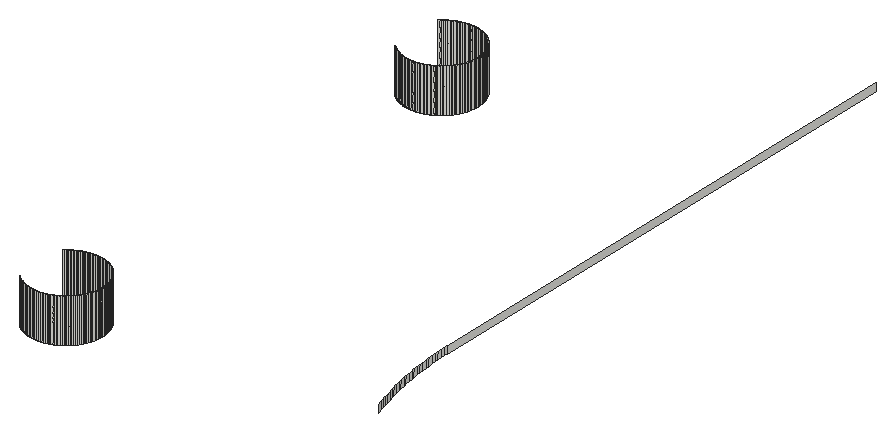
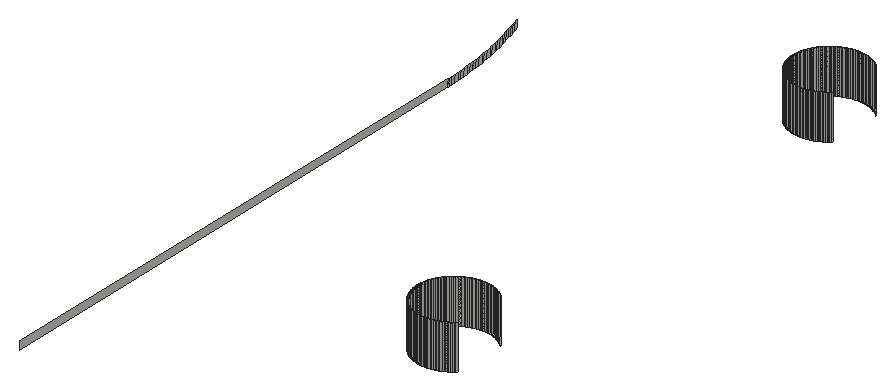
# SketchUp Ruby script. Lengths in inches.
U = 1.inch
M = Sketchup.active_model
def pt(a) = Geom::Point3d.new(a.map { |v| v * U })
def face(e, loops, mat)
  f = e.add_face(loops[0].map { |a| pt(a) })
  loops[1..].each { |l| e.add_face(l.map { |a| pt(a) }).erase! }
  f.material = f.back_material = mat if mat
  f
end
# faces: each face lists its corners as indices into pts; further lists are holes
def faces(e, pts, list, mat = nil) = list.each { |f| face(e, (f[0].is_a?(Array) ? f : [f]).map { |l| l.map { |i| pts[i] } }, mat) }
# xy, xz, yz: faces in a plane at the given z, y or x. An outline is a flat list of corners, or four numbers for a rectangle; further outlines are holes
def ring(l) = l.size == 4 ? [[l[0], l[1]], [l[2], l[1]], [l[2], l[3]], [l[0], l[3]]] : l.each_slice(2).to_a
def flat(e, list, mat, &to3) = list.each { |f| face(e, (f[0].is_a?(Array) ? f : [f]).map { |l| ring(l).map { |u, v| to3.(u, v) } }, mat) }
def xy(e, z, list, mat = nil) = flat(e, list, mat) { |x, y| [x, y, z] }
def xz(e, y, list, mat = nil) = flat(e, list, mat) { |x, z| [x, y, z] }
def yz(e, x, list, mat = nil) = flat(e, list, mat) { |y, z| [x, y, z] }
def lines(e, pts, list) = list.each { |a, b| e.add_line(pt(pts[a]), pt(pts[b])) }
# prism: a flat outline (further loops are holes) pulled along v
def prism(e, loops, v, mat = nil)
  f = face(e, loops, mat); d = Geom::Vector3d.new(v.map { |x| x * U })
  f.pushpull(f.normal.samedirection?(d) ? d.length : -d.length)
end
def box(e, o, s, mat = nil) = prism(e, [[o, [o[0] + s[0], o[1], o[2]], [o[0] + s[0], o[1] + s[1], o[2]], [o[0], o[1] + s[1], o[2]]]], [0, 0, s[2]], mat)
def at(x, y, z, deg = 0) = Geom::Transformation.translation(pt([x, y, z])) * Geom::Transformation.rotation(ORIGIN, Z_AXIS, deg.degrees)
def axes(o, x, y, z) = Geom::Transformation.new([*x, 0, *y, 0, *z, 0, *pt(o).to_a, 1])
def part(name) = M.definitions.add(name)
# library, detail: a bought-in or finely detailed component or shape, given as its bounding box
def library(name, o, s) = part(name).tap { |d| box(d.entities, o, s) }
def detail(e, o, s) = box(e.add_group.entities, o, s)
def put(e, d, t, mat = nil) = e.add_instance(d, t).tap { |i| i.material = mat if mat }
def group(e, t, mat = nil) = e.add_group.tap { |g| g.transformation = t; g.material = mat if mat }.entities
root = M.entities
xz(root,197.5,[[110.34,116,110.42,119],[110.42,116,110.5,119],[110.5,116,110.58,119],[110.58,116,110.66,119]])
xz(root,202.5,[[110.34,116,110.42,119],[110.42,116,110.5,119],[110.5,116,110.58,119],[110.58,116,110.66,119]])
xz(root,229.5,[[110.34,116,110.42,119],[110.42,116,110.5,119],[110.5,116,110.58,119],[110.58,116,110.66,119]])
xz(root,234.5,[[110.34,116,110.42,119],[110.42,116,110.5,119],[110.5,116,110.58,119],[110.58,116,110.66,119]])
yz(root,113,[[199.84,116,199.92,119],[199.92,116,200,119],[200,116,200.08,119],[200.08,116,200.16,119],[231.84,116,231.92,119],
  [231.92,116,232,119],[232,116,232.08,119],[232.08,116,232.16,119]])
yz(root,128.5,[[209.72,116,209.95,116.5],[209.95,116,209.99,116.5],[209.99,116,246.5,116.5]])
p = [[110.03,197.54,116],[109.95,197.56,116],[109.95,197.56,119],[110.03,197.54,119],[110.11,197.53,116],[110.11,197.53,119],
  [110.1875,197.52,116],[110.1875,197.52,119],[110.26,197.51,116],[110.26,197.51,119],[110.34,197.5,116],[110.34,197.5,119],
  [110.74,197.51,116],[110.66,197.5,116],[110.66,197.5,119],[110.74,197.51,119],[110.8125,197.52,116],[110.8125,197.52,119],
  [110.89,197.53,116],[110.89,197.53,119],[110.97,197.54,116],[110.97,197.54,119],[111.05,197.56,116],[111.05,197.56,119],
  [109.65,197.65,116],[109.58,197.68,116],[109.58,197.68,119],[109.65,197.65,119],[109.73,197.62,116],[109.73,197.62,119],
  [109.8,197.6,116],[109.8,197.6,119],[109.88,197.58,116],[109.88,197.58,119],[111.12,197.58,116],[111.12,197.58,119],
  [111.2,197.6,116],[111.2,197.6,119],[111.27,197.62,116],[111.27,197.62,119],[111.35,197.65,116],[111.35,197.65,119],
  [111.42,197.68,116],[111.42,197.68,119],[109.4375,197.74,116],[109.37,197.77,116],[109.37,197.77,119],[109.4375,197.74,119],
  [109.51,197.71,116],[109.51,197.71,119],[111.49,197.71,116],[111.49,197.71,119],[111.5625,197.74,116],[111.5625,197.74,119],
  [111.63,197.77,116],[111.63,197.77,119],[109.23,197.85,116],[109.16,197.89,116],[109.16,197.89,119],[109.23,197.85,119],
  [109.3,197.81,116],[109.3,197.81,119],[111.7,197.81,116],[111.7,197.81,119],[111.77,197.85,116],[111.77,197.85,119],
  [111.84,197.89,116],[111.84,197.89,119],[109.09,197.93,116],[109.03,197.98,116],[109.03,197.98,119],[109.09,197.93,119],
  [111.91,197.93,116],[111.91,197.93,119],[111.97,197.98,116],[111.97,197.98,119],[108.97,198.02,116],[108.91,198.07,116],
  [108.91,198.07,119],[108.97,198.02,119],[112.03,198.02,116],[112.03,198.02,119],[112.09,198.07,116],[112.09,198.07,119],
  [108.85,198.125,116],[108.79,198.18,116],[108.79,198.18,119],[108.85,198.125,119],[112.15,198.125,116],[112.15,198.125,119],
  [112.21,198.18,116],[112.21,198.18,119],[112.27,198.23,116],[112.27,198.23,119],[112.32,198.29,116],[112.32,198.29,119],
  [112.375,198.35,116],[112.375,198.35,119],[112.43,198.41,116],[112.43,198.41,119],[112.48,198.47,116],[112.48,198.47,119],
  [112.52,198.53,116],[112.52,198.53,119],[112.57,198.59,116],[112.57,198.59,119],[112.61,198.66,116],[112.61,198.66,119],
  [112.65,198.73,116],[112.65,198.73,119],[112.69,198.8,116],[112.69,198.8,119],[112.73,198.87,116],[112.73,198.87,119],
  [112.76,198.9375,116],[112.76,198.9375,119],[112.79,199.01,116],[112.79,199.01,119],[112.82,199.08,116],[112.82,199.08,119],
  [112.85,199.15,116],[112.85,199.15,119],[112.88,199.23,116],[112.88,199.23,119],[112.9,199.3,116],[112.9,199.3,119],
  [112.92,199.38,116],[112.92,199.38,119],[112.94,199.45,116],[112.94,199.45,119],[112.96,199.53,116],[112.96,199.53,119],
  [112.97,199.61,116],[112.97,199.61,119],[112.98,199.6875,116],[112.98,199.6875,119],[112.99,199.76,116],[112.99,199.76,119],
  [113,199.84,116],[113,199.84,119],[112.98,200.3125,116],[112.99,200.24,116],[112.99,200.24,119],[112.98,200.3125,119],
  [113,200.16,116],[113,200.16,119],[112.97,200.39,116],[112.97,200.39,119],[112.96,200.47,116],[112.96,200.47,119],
  [112.92,200.62,116],[112.94,200.55,116],[112.94,200.55,119],[112.92,200.62,119],[112.9,200.7,116],[112.9,200.7,119],
  [112.88,200.77,116],[112.88,200.77,119],[112.82,200.92,116],[112.85,200.85,116],[112.85,200.85,119],[112.82,200.92,119],
  [112.79,200.99,116],[112.79,200.99,119],[112.76,201.0625,116],[112.76,201.0625,119],[112.69,201.2,116],[112.73,201.13,116],
  [112.73,201.13,119],[112.69,201.2,119],[112.65,201.27,116],[112.65,201.27,119],[112.57,201.41,116],[112.61,201.34,116],
  [112.61,201.34,119],[112.57,201.41,119],[112.52,201.47,116],[112.52,201.47,119],[112.43,201.59,116],[112.48,201.53,116],
  [112.48,201.53,119],[112.43,201.59,119],[112.375,201.65,116],[112.375,201.65,119],[112.27,201.77,116],[112.32,201.71,116],
  [112.32,201.71,119],[112.27,201.77,119],[108.79,201.82,116],[108.85,201.875,116],[108.85,201.875,119],[108.79,201.82,119],
  [112.15,201.875,116],[112.21,201.82,116],[112.21,201.82,119],[112.15,201.875,119],[108.91,201.93,116],[108.91,201.93,119],
  [108.97,201.98,116],[108.97,201.98,119],[112.03,201.98,116],[112.09,201.93,116],[112.09,201.93,119],[112.03,201.98,119],
  [109.03,202.02,116],[109.03,202.02,119],[109.09,202.07,116],[109.09,202.07,119],[111.91,202.07,116],[111.97,202.02,116],
  [111.97,202.02,119],[111.91,202.07,119],[109.16,202.11,116],[109.16,202.11,119],[109.23,202.15,116],[109.23,202.15,119],
  [111.77,202.15,116],[111.84,202.11,116],[111.84,202.11,119],[111.77,202.15,119],[109.3,202.19,116],[109.3,202.19,119],
  [109.37,202.23,116],[109.37,202.23,119],[109.4375,202.26,116],[109.4375,202.26,119],[111.5625,202.26,116],[111.63,202.23,116],
  [111.63,202.23,119],[111.5625,202.26,119],[111.7,202.19,116],[111.7,202.19,119],[109.51,202.29,116],[109.51,202.29,119],
  [109.58,202.32,116],[109.58,202.32,119],[109.65,202.35,116],[109.65,202.35,119],[111.35,202.35,116],[111.42,202.32,116],
  [111.42,202.32,119],[111.35,202.35,119],[111.49,202.29,116],[111.49,202.29,119],[109.73,202.38,116],[109.73,202.38,119],
  [109.8,202.4,116],[109.8,202.4,119],[109.88,202.42,116],[109.88,202.42,119],[109.95,202.44,116],[109.95,202.44,119],
  [110.03,202.46,116],[110.03,202.46,119],[110.97,202.46,116],[111.05,202.44,116],[111.05,202.44,119],[110.97,202.46,119],
  [111.12,202.42,116],[111.12,202.42,119],[111.2,202.4,116],[111.2,202.4,119],[111.27,202.38,116],[111.27,202.38,119],
  [110.11,202.47,116],[110.11,202.47,119],[110.1875,202.48,116],[110.1875,202.48,119],[110.26,202.49,116],[110.26,202.49,119],
  [110.34,202.5,116],[110.34,202.5,119],[110.66,202.5,116],[110.74,202.49,116],[110.74,202.49,119],[110.66,202.5,119],
  [110.8125,202.48,116],[110.8125,202.48,119],[110.89,202.47,116],[110.89,202.47,119],[129.65,202.74,116],[129.5625,203.01,116],
  [129.5625,203.01,116.5],[129.65,202.74,116.5],[129.48,203.28,116],[129.48,203.28,116.5],[129.4,203.55,116],[129.4,203.55,116.5],
  [129.33,203.83,116],[129.33,203.83,116.5],[129.25,204.1,116],[129.25,204.1,116.5],[129.18,204.375,116],[129.18,204.375,116.5],
  [129.12,204.65,116],[129.12,204.65,116.5],[129.05,204.93,116],[129.05,204.93,116.5],[128.99,205.21,116],[128.99,205.21,116.5],
  [128.9375,205.49,116],[128.9375,205.49,116.5],[128.88,205.76,116],[128.88,205.76,116.5],[128.84,206.04,116],[128.84,206.04,116.5],
  [128.79,206.32,116],[128.79,206.32,116.5],[128.75,206.6,116],[128.75,206.6,116.5],[128.71,206.89,116],[128.71,206.89,116.5],
  [128.67,207.17,116],[128.67,207.17,116.5],[128.64,207.45,116],[128.64,207.45,116.5],[128.61,207.73,116],[128.61,207.73,116.5],
  [128.58,208.01,116],[128.58,208.01,116.5],[128.5625,208.3,116],[128.5625,208.3,116.5],[128.54,208.58,116],[128.54,208.58,116.5],
  [128.53,208.86,116],[128.53,208.86,116.5],[128.52,209.15,116],[128.52,209.15,116.5],[128.51,209.43,116],[128.51,209.43,116.5],
  [128.5,209.72,116],[128.5,209.72,116.5],[110.03,229.54,116],[109.95,229.56,116],[109.95,229.56,119],[110.03,229.54,119],
  [110.11,229.53,116],[110.11,229.53,119],[110.1875,229.52,116],[110.1875,229.52,119],[110.26,229.51,116],[110.26,229.51,119],
  [110.34,229.5,116],[110.34,229.5,119],[110.74,229.51,116],[110.66,229.5,116],[110.66,229.5,119],[110.74,229.51,119],
  [110.8125,229.52,116],[110.8125,229.52,119],[110.89,229.53,116],[110.89,229.53,119],[110.97,229.54,116],[110.97,229.54,119],
  [111.05,229.56,116],[111.05,229.56,119],[109.65,229.65,116],[109.58,229.68,116],[109.58,229.68,119],[109.65,229.65,119],
  [109.73,229.62,116],[109.73,229.62,119],[109.8,229.6,116],[109.8,229.6,119],[109.88,229.58,116],[109.88,229.58,119],
  [111.12,229.58,116],[111.12,229.58,119],[111.2,229.6,116],[111.2,229.6,119],[111.27,229.62,116],[111.27,229.62,119],
  [111.35,229.65,116],[111.35,229.65,119],[111.42,229.68,116],[111.42,229.68,119],[109.4375,229.74,116],[109.37,229.77,116],
  [109.37,229.77,119],[109.4375,229.74,119],[109.51,229.71,116],[109.51,229.71,119],[111.49,229.71,116],[111.49,229.71,119],
  [111.5625,229.74,116],[111.5625,229.74,119],[111.63,229.77,116],[111.63,229.77,119],[109.23,229.85,116],[109.16,229.89,116],
  [109.16,229.89,119],[109.23,229.85,119],[109.3,229.81,116],[109.3,229.81,119],[111.7,229.81,116],[111.7,229.81,119],
  [111.77,229.85,116],[111.77,229.85,119],[111.84,229.89,116],[111.84,229.89,119],[109.09,229.93,116],[109.03,229.98,116],
  [109.03,229.98,119],[109.09,229.93,119],[111.91,229.93,116],[111.91,229.93,119],[111.97,229.98,116],[111.97,229.98,119],
  [108.97,230.02,116],[108.91,230.07,116],[108.91,230.07,119],[108.97,230.02,119],[112.03,230.02,116],[112.03,230.02,119],
  [112.09,230.07,116],[112.09,230.07,119],[108.85,230.125,116],[108.79,230.18,116],[108.79,230.18,119],[108.85,230.125,119],
  [112.15,230.125,116],[112.15,230.125,119],[112.21,230.18,116],[112.21,230.18,119],[112.27,230.23,116],[112.27,230.23,119],
  [112.32,230.29,116],[112.32,230.29,119],[112.375,230.35,116],[112.375,230.35,119],[112.43,230.41,116],[112.43,230.41,119],
  [112.48,230.47,116],[112.48,230.47,119],[112.52,230.53,116],[112.52,230.53,119],[112.57,230.59,116],[112.57,230.59,119],
  [112.61,230.66,116],[112.61,230.66,119],[112.65,230.73,116],[112.65,230.73,119],[112.69,230.8,116],[112.69,230.8,119],
  [112.73,230.87,116],[112.73,230.87,119],[112.76,230.9375,116],[112.76,230.9375,119],[112.79,231.01,116],[112.79,231.01,119],
  [112.82,231.08,116],[112.82,231.08,119],[112.85,231.15,116],[112.85,231.15,119],[112.88,231.23,116],[112.88,231.23,119],
  [112.9,231.3,116],[112.9,231.3,119],[112.92,231.38,116],[112.92,231.38,119],[112.94,231.45,116],[112.94,231.45,119],
  [112.96,231.53,116],[112.96,231.53,119],[112.97,231.61,116],[112.97,231.61,119],[112.98,231.6875,116],[112.98,231.6875,119],
  [112.99,231.76,116],[112.99,231.76,119],[113,231.84,116],[113,231.84,119],[112.98,232.3125,116],[112.99,232.24,116],
  [112.99,232.24,119],[112.98,232.3125,119],[113,232.16,116],[113,232.16,119],[112.97,232.39,116],[112.97,232.39,119],
  [112.96,232.47,116],[112.96,232.47,119],[112.92,232.62,116],[112.94,232.55,116],[112.94,232.55,119],[112.92,232.62,119],
  [112.9,232.7,116],[112.9,232.7,119],[112.88,232.77,116],[112.88,232.77,119],[112.82,232.92,116],[112.85,232.85,116],
  [112.85,232.85,119],[112.82,232.92,119],[112.79,232.99,116],[112.79,232.99,119],[112.76,233.0625,116],[112.76,233.0625,119],
  [112.69,233.2,116],[112.73,233.13,116],[112.73,233.13,119],[112.69,233.2,119],[112.65,233.27,116],[112.65,233.27,119],
  [112.57,233.41,116],[112.61,233.34,116],[112.61,233.34,119],[112.57,233.41,119],[112.52,233.47,116],[112.52,233.47,119],
  [112.43,233.59,116],[112.48,233.53,116],[112.48,233.53,119],[112.43,233.59,119],[112.375,233.65,116],[112.375,233.65,119],
  [112.27,233.77,116],[112.32,233.71,116],[112.32,233.71,119],[112.27,233.77,119],[108.79,233.82,116],[108.85,233.875,116],
  [108.85,233.875,119],[108.79,233.82,119],[112.15,233.875,116],[112.21,233.82,116],[112.21,233.82,119],[112.15,233.875,119],
  [108.91,233.93,116],[108.91,233.93,119],[108.97,233.98,116],[108.97,233.98,119],[112.03,233.98,116],[112.09,233.93,116],
  [112.09,233.93,119],[112.03,233.98,119],[109.03,234.02,116],[109.03,234.02,119],[109.09,234.07,116],[109.09,234.07,119],
  [111.91,234.07,116],[111.97,234.02,116],[111.97,234.02,119],[111.91,234.07,119],[109.16,234.11,116],[109.16,234.11,119],
  [109.23,234.15,116],[109.23,234.15,119],[111.77,234.15,116],[111.84,234.11,116],[111.84,234.11,119],[111.77,234.15,119],
  [109.3,234.19,116],[109.3,234.19,119],[109.37,234.23,116],[109.37,234.23,119],[109.4375,234.26,116],[109.4375,234.26,119],
  [111.5625,234.26,116],[111.63,234.23,116],[111.63,234.23,119],[111.5625,234.26,119],[111.7,234.19,116],[111.7,234.19,119],
  [109.51,234.29,116],[109.51,234.29,119],[109.58,234.32,116],[109.58,234.32,119],[109.65,234.35,116],[109.65,234.35,119],
  [111.35,234.35,116],[111.42,234.32,116],[111.42,234.32,119],[111.35,234.35,119],[111.49,234.29,116],[111.49,234.29,119],
  [109.73,234.38,116],[109.73,234.38,119],[109.8,234.4,116],[109.8,234.4,119],[109.88,234.42,116],[109.88,234.42,119],
  [109.95,234.44,116],[109.95,234.44,119],[110.03,234.46,116],[110.03,234.46,119],[110.97,234.46,116],[111.05,234.44,116],
  [111.05,234.44,119],[110.97,234.46,119],[111.12,234.42,116],[111.12,234.42,119],[111.2,234.4,116],[111.2,234.4,119],
  [111.27,234.38,116],[111.27,234.38,119],[110.11,234.47,116],[110.11,234.47,119],[110.1875,234.48,116],[110.1875,234.48,119],
  [110.26,234.49,116],[110.26,234.49,119],[110.34,234.5,116],[110.34,234.5,119],[110.66,234.5,116],[110.74,234.49,116],
  [110.74,234.49,119],[110.66,234.5,119],[110.8125,234.48,116],[110.8125,234.48,119],[110.89,234.47,116],[110.89,234.47,119]]
faces(root,p,[[0,1,2,3],[4,0,3,5],[6,4,5,7],[8,6,7,9],[10,8,9,11],[12,13,14,15],[16,12,15,17],[18,16,17,19],
  [20,18,19,21],[22,20,21,23],[24,25,26,27],[28,24,27,29],[30,28,29,31],[32,30,31,33],[1,32,33,2],[34,22,23,35],
  [36,34,35,37],[38,36,37,39],[40,38,39,41],[42,40,41,43],[44,45,46,47],[48,44,47,49],[25,48,49,26],[50,42,43,51],
  [52,50,51,53],[54,52,53,55],[56,57,58,59],[60,56,59,61],[45,60,61,46],[62,54,55,63],[64,62,63,65],[66,64,65,67],
  [68,69,70,71],[57,68,71,58],[72,66,67,73],[74,72,73,75],[76,77,78,79],[69,76,79,70],[80,74,75,81],[82,80,81,83],
  [84,85,86,87],[77,84,87,78],[88,82,83,89],[90,88,89,91],[92,90,91,93],[94,92,93,95],[96,94,95,97],[98,96,97,99],
  [100,98,99,101],[102,100,101,103],[104,102,103,105],[106,104,105,107],[108,106,107,109],[110,108,109,111],[112,110,111,113],[114,112,113,115],
  [116,114,115,117],[118,116,117,119],[120,118,119,121],[122,120,121,123],[124,122,123,125],[126,124,125,127],[128,126,127,129],[130,128,129,131],
  [132,130,131,133],[134,132,133,135],[136,134,135,137],[138,136,137,139],[140,141,142,143],[141,144,145,142],[146,140,143,147],[148,146,147,149],
  [150,151,152,153],[151,148,149,152],[154,150,153,155],[156,154,155,157],[158,159,160,161],[159,156,157,160],[162,158,161,163],[164,162,163,165],
  [166,167,168,169],[167,164,165,168],[170,166,169,171],[172,173,174,175],[173,170,171,174],[176,172,175,177],[178,179,180,181],[179,176,177,180],
  [182,178,181,183],[184,185,186,187],[185,182,183,186],[188,189,190,191],[192,193,194,195],[193,184,187,194],[189,196,197,190],[196,198,199,197],
  [200,201,202,203],[201,192,195,202],[198,204,205,199],[204,206,207,205],[208,209,210,211],[209,200,203,210],[206,212,213,207],[212,214,215,213],
  [216,217,218,219],[217,208,211,218],[214,220,221,215],[220,222,223,221],[222,224,225,223],[226,227,228,229],[227,230,231,228],[230,216,219,231],
  [224,232,233,225],[232,234,235,233],[234,236,237,235],[238,239,240,241],[239,242,243,240],[242,226,229,243],[236,244,245,237],[244,246,247,245],
  [246,248,249,247],[248,250,251,249],[250,252,253,251],[254,255,256,257],[255,258,259,256],[258,260,261,259],[260,262,263,261],[262,238,241,263],
  [252,264,265,253],[264,266,267,265],[266,268,269,267],[268,270,271,269],[272,273,274,275],[273,276,277,274],[276,278,279,277],[278,254,257,279],
  [280,281,282,283],[281,284,285,282],[284,286,287,285],[286,288,289,287],[288,290,291,289],[290,292,293,291],[292,294,295,293],[294,296,297,295],
  [296,298,299,297],[298,300,301,299],[300,302,303,301],[302,304,305,303],[304,306,307,305],[306,308,309,307],[308,310,311,309],[310,312,313,311],
  [312,314,315,313],[314,316,317,315],[316,318,319,317],[318,320,321,319],[320,322,323,321],[322,324,325,323],[324,326,327,325],[326,328,329,327],
  [328,330,331,329],[332,333,334,335],[336,332,335,337],[338,336,337,339],[340,338,339,341],[342,340,341,343],[344,345,346,347],[348,344,347,349],
  [350,348,349,351],[352,350,351,353],[354,352,353,355],[356,357,358,359],[360,356,359,361],[362,360,361,363],[364,362,363,365],[333,364,365,334],
  [366,354,355,367],[368,366,367,369],[370,368,369,371],[372,370,371,373],[374,372,373,375],[376,377,378,379],[380,376,379,381],[357,380,381,358],
  [382,374,375,383],[384,382,383,385],[386,384,385,387],[388,389,390,391],[392,388,391,393],[377,392,393,378],[394,386,387,395],[396,394,395,397],
  [398,396,397,399],[400,401,402,403],[389,400,403,390],[404,398,399,405],[406,404,405,407],[408,409,410,411],[401,408,411,402],[412,406,407,413],
  [414,412,413,415],[416,417,418,419],[409,416,419,410],[420,414,415,421],[422,420,421,423],[424,422,423,425],[426,424,425,427],[428,426,427,429],
  [430,428,429,431],[432,430,431,433],[434,432,433,435],[436,434,435,437],[438,436,437,439],[440,438,439,441],[442,440,441,443],[444,442,443,445],
  [446,444,445,447],[448,446,447,449],[450,448,449,451],[452,450,451,453],[454,452,453,455],[456,454,455,457],[458,456,457,459],[460,458,459,461],
  [462,460,461,463],[464,462,463,465],[466,464,465,467],[468,466,467,469],[470,468,469,471],[472,473,474,475],[473,476,477,474],[478,472,475,479],
  [480,478,479,481],[482,483,484,485],[483,480,481,484],[486,482,485,487],[488,486,487,489],[490,491,492,493],[491,488,489,492],[494,490,493,495],
  [496,494,495,497],[498,499,500,501],[499,496,497,500],[502,498,501,503],[504,505,506,507],[505,502,503,506],[508,504,507,509],[510,511,512,513],
  [511,508,509,512],[514,510,513,515],[516,517,518,519],[517,514,515,518],[520,521,522,523],[524,525,526,527],[525,516,519,526],[521,528,529,522],
  [528,530,531,529],[532,533,534,535],[533,524,527,534],[530,536,537,531],[536,538,539,537],[540,541,542,543],[541,532,535,542],[538,544,545,539],
  [544,546,547,545],[548,549,550,551],[549,540,543,550],[546,552,553,547],[552,554,555,553],[554,556,557,555],[558,559,560,561],[559,562,563,560],
  [562,548,551,563],[556,564,565,557],[564,566,567,565],[566,568,569,567],[570,571,572,573],[571,574,575,572],[574,558,561,575],[568,576,577,569],
  [576,578,579,577],[578,580,581,579],[580,582,583,581],[582,584,585,583],[586,587,588,589],[587,590,591,588],[590,592,593,591],[592,594,595,593],
  [594,570,573,595],[584,596,597,585],[596,598,599,597],[598,600,601,599],[600,602,603,601],[604,605,606,607],[605,608,609,606],[608,610,611,609],
  [610,586,589,611]])
